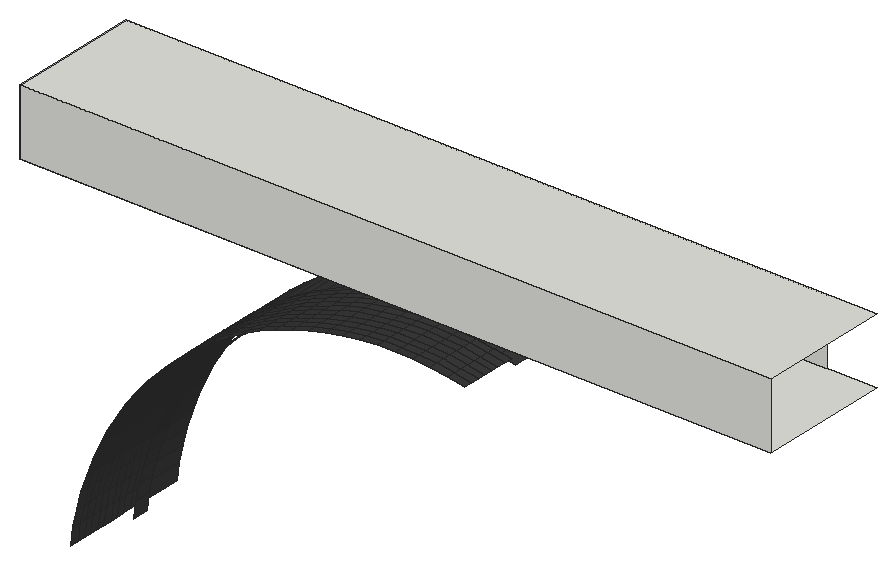
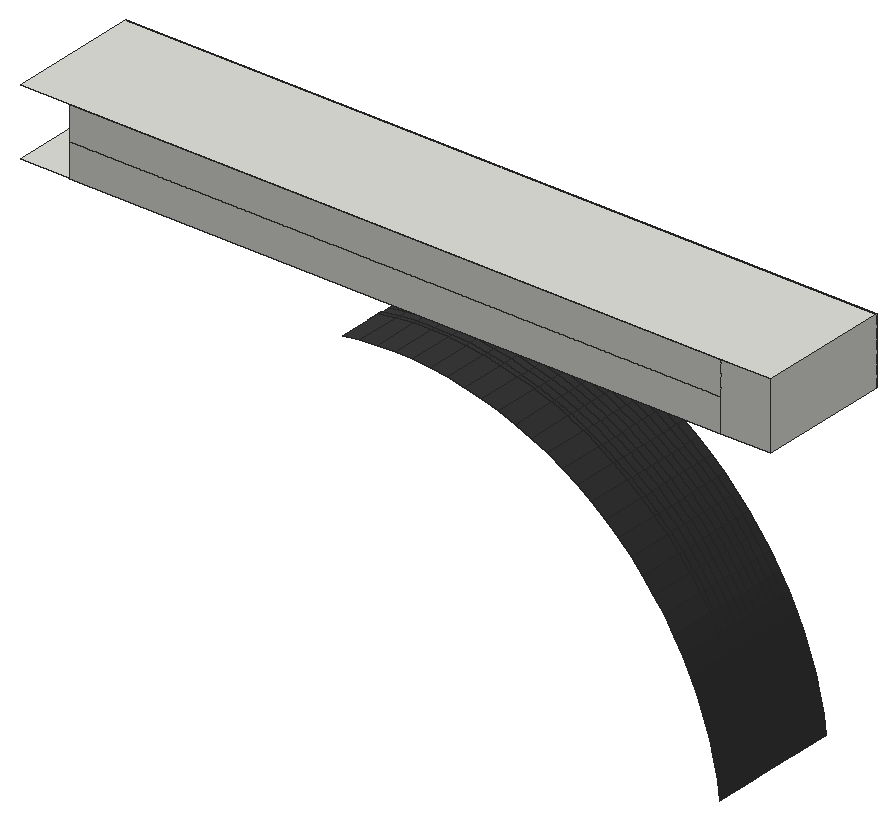
# SketchUp Ruby script. Lengths in inches.
U = 1.inch
M = Sketchup.active_model
def pt(a) = Geom::Point3d.new(a.map { |v| v * U })
def face(e, loops, mat)
  f = e.add_face(loops[0].map { |a| pt(a) })
  loops[1..].each { |l| e.add_face(l.map { |a| pt(a) }).erase! }
  f.material = f.back_material = mat if mat
  f
end
# faces: each face lists its corners as indices into pts; further lists are holes
def faces(e, pts, list, mat = nil) = list.each { |f| face(e, (f[0].is_a?(Array) ? f : [f]).map { |l| l.map { |i| pts[i] } }, mat) }
# xy, xz, yz: faces in a plane at the given z, y or x. An outline is a flat list of corners, or four numbers for a rectangle; further outlines are holes
def ring(l) = l.size == 4 ? [[l[0], l[1]], [l[2], l[1]], [l[2], l[3]], [l[0], l[3]]] : l.each_slice(2).to_a
def flat(e, list, mat, &to3) = list.each { |f| face(e, (f[0].is_a?(Array) ? f : [f]).map { |l| ring(l).map { |u, v| to3.(u, v) } }, mat) }
def xy(e, z, list, mat = nil) = flat(e, list, mat) { |x, y| [x, y, z] }
def xz(e, y, list, mat = nil) = flat(e, list, mat) { |x, z| [x, y, z] }
def yz(e, x, list, mat = nil) = flat(e, list, mat) { |y, z| [x, y, z] }
def lines(e, pts, list) = list.each { |a, b| e.add_line(pt(pts[a]), pt(pts[b])) }
# prism: a flat outline (further loops are holes) pulled along v
def prism(e, loops, v, mat = nil)
  f = face(e, loops, mat); d = Geom::Vector3d.new(v.map { |x| x * U })
  f.pushpull(f.normal.samedirection?(d) ? d.length : -d.length)
end
def box(e, o, s, mat = nil) = prism(e, [[o, [o[0] + s[0], o[1], o[2]], [o[0] + s[0], o[1] + s[1], o[2]], [o[0], o[1] + s[1], o[2]]]], [0, 0, s[2]], mat)
def at(x, y, z, deg = 0) = Geom::Transformation.translation(pt([x, y, z])) * Geom::Transformation.rotation(ORIGIN, Z_AXIS, deg.degrees)
def axes(o, x, y, z) = Geom::Transformation.new([*x, 0, *y, 0, *z, 0, *pt(o).to_a, 1])
def part(name) = M.definitions.add(name)
# library, detail: a bought-in or finely detailed component or shape, given as its bounding box
def library(name, o, s) = part(name).tap { |d| box(d.entities, o, s) }
def detail(e, o, s) = box(e.add_group.entities, o, s)
def put(e, d, t, mat = nil) = e.add_instance(d, t).tap { |i| i.material = mat if mat }
def group(e, t, mat = nil) = e.add_group.tap { |g| g.transformation = t; g.material = mat if mat }.entities
root = M.entities
M.materials.add("[Color M07]").color = [58, 58, 58]
xy(root,373.6875,[[18.46,0,154.46,24]])
xy(root,385.6875,[[18.46,0,154.46,24]])
xz(root,0,[[18.46,373.6875,154.46,385.6875]])
xz(root,24,[[18.46,373.6875,27.46,385.6875],[27.46,373.6875,145.46,379.6875],[27.46,379.6875,145.46,385.6875]])
yz(root,18.46,[[0,373.6875,24,385.6875]])
p = [[29.42,14.875,313.82],[29.87,14.875,316.87],[29.87,12,316.87],[29.42,12,313.82],[27.6,0,314.03],[27.6,1.5,314.03],
  [28.06,1.5,317.1875],[28.06,0,317.1875],[27.6,3,314.03],[28.06,3,317.1875],[27.6,4.5,314.03],[28.06,4.5,317.1875],
  [27.6,6,314.03],[28.06,6,317.1875],[27.6,7.5,314.03],[28.06,7.5,317.1875],[27.6,9,314.03],[28.06,9,317.1875],
  [27.6,10.5,314.03],[28.06,10.5,317.1875],[27.6,12,314.03],[28.06,12,317.1875],[27.6,13.5,314.03],[28.06,13.5,317.1875],
  [27.6,15,314.03],[28.06,15,317.1875],[27.6,15.8125,314.03],[28.06,15.8125,317.1875],[28.06,24,317.1875],[27.6,24,314.03],
  [30.48,14.875,319.9],[30.48,12,319.9],[28.7,1.5,320.31],[28.7,0,320.31],[28.7,3,320.31],[28.7,4.5,320.31],
  [28.7,6,320.31],[28.7,7.5,320.31],[28.7,9,320.31],[28.7,10.5,320.31],[28.7,12,320.31],[28.7,13.5,320.31],
  [28.7,15,320.31],[28.7,15.8125,320.31],[28.7,24,320.31],[31.26,14.875,322.89],[31.26,12,322.89],[29.5,1.5,323.39],
  [29.5,0,323.39],[29.5,3,323.39],[29.5,4.5,323.39],[29.5,6,323.39],[29.5,7.5,323.39],[29.5,9,323.39],
  [29.5,10.5,323.39],[29.5,12,323.39],[29.5,13.5,323.39],[29.5,15,323.39],[29.5,15.8125,323.39],[29.5,24,323.39],
  [32.19,14.875,325.83],[32.19,12,325.83],[30.46,1.5,326.43],[30.46,0,326.43],[30.46,3,326.43],[30.46,4.5,326.43],
  [30.46,6,326.43],[30.46,7.5,326.43],[30.46,9,326.43],[30.46,10.5,326.43],[30.46,12,326.43],[30.46,13.5,326.43],
  [30.46,15,326.43],[30.46,15.8125,326.43],[30.46,24,326.43],[33.28,14.875,328.72],[33.28,12,328.72],[31.59,1.5,329.41],
  [31.59,0,329.41],[31.59,3,329.41],[31.59,4.5,329.41],[31.59,6,329.41],[31.59,7.5,329.41],[31.59,9,329.41],
  [31.59,10.5,329.41],[31.59,12,329.41],[31.59,13.5,329.41],[31.59,15,329.41],[31.59,15.8125,329.41],[31.59,24,329.41],
  [34.53,14.875,331.54],[34.53,12,331.54],[32.875,1.5,332.33],[32.875,0,332.33],[32.875,3,332.33],[32.875,4.5,332.33],
  [32.875,6,332.33],[32.875,7.5,332.33],[32.875,9,332.33],[32.875,10.5,332.33],[32.875,12,332.33],[32.875,13.5,332.33],
  [32.875,15,332.33],[32.875,15.8125,332.33],[32.875,24,332.33],[35.92,14.875,334.3],[35.92,12,334.3],[34.3125,1.5,335.17],
  [34.3125,0,335.17],[34.3125,3,335.17],[34.3125,4.5,335.17],[34.3125,6,335.17],[34.3125,7.5,335.17],[34.3125,9,335.17],
  [34.3125,10.5,335.17],[34.3125,12,335.17],[34.3125,13.5,335.17],[34.3125,15,335.17],[34.3125,15.8125,335.17],[34.3125,24,335.17],
  [37.47,14.875,336.97],[37.47,12,336.97],[35.9,1.5,337.93],[35.9,0,337.93],[35.9,3,337.93],[35.9,4.5,337.93],
  [35.9,6,337.93],[35.9,7.5,337.93],[35.9,9,337.93],[35.9,10.5,337.93],[35.9,12,337.93],[35.9,13.5,337.93],
  [35.9,15,337.93],[35.9,15.8125,337.93],[35.9,24,337.93],[39.15,14.875,339.5625],[39.15,12,339.5625],[37.64,1.5,340.6],
  [37.64,0,340.6],[37.64,3,340.6],[37.64,4.5,340.6],[37.64,6,340.6],[37.64,7.5,340.6],[37.64,9,340.6],
  [37.64,10.5,340.6],[37.64,12,340.6],[37.64,13.5,340.6],[37.64,15,340.6],[37.64,15.8125,340.6],[37.64,24,340.6],
  [40.97,14.875,342.06],[40.97,12,342.06],[39.52,1.5,343.17],[39.52,0,343.17],[39.52,3,343.17],[39.52,4.5,343.17],
  [39.52,6,343.17],[39.52,7.5,343.17],[39.52,9,343.17],[39.52,10.5,343.17],[39.52,12,343.17],[39.52,13.5,343.17],
  [39.52,15,343.17],[39.52,15.8125,343.17],[39.52,24,343.17],[42.92,14.875,344.45],[42.92,12,344.45],[41.53,1.5,345.64],
  [41.53,0,345.64],[41.53,3,345.64],[41.53,4.5,345.64],[41.53,6,345.64],[41.53,7.5,345.64],[41.53,9,345.64],
  [41.53,10.5,345.64],[41.53,12,345.64],[41.53,13.5,345.64],[41.53,15,345.64],[41.53,15.8125,345.64],[41.53,24,345.64],
  [45,14.875,346.74],[45,12,346.74],[43.67,1.5,348],[43.67,0,348],[43.67,3,348],[43.67,4.5,348],
  [43.67,6,348],[43.67,7.5,348],[43.67,9,348],[43.67,10.5,348],[43.67,12,348],[43.67,13.5,348],
  [43.67,15,348],[43.67,15.8125,348],[43.67,24,348],[47.19,14.875,348.91],[47.19,12,348.91],[45.94,1.5,350.24],
  [45.94,0,350.24],[45.94,3,350.24],[45.94,4.5,350.24],[45.94,6,350.24],[45.94,7.5,350.24],[45.94,9,350.24],
  [45.94,10.5,350.24],[45.94,12,350.24],[45.94,13.5,350.24],[45.94,15,350.24],[45.94,15.8125,350.24],[45.94,24,350.24],
  [48.35,14.875,349.93],[49.5,14.875,350.95],[49.5,12,350.95],[48.35,12,349.93],[48.32,1.5,352.36],[48.32,0,352.36],
  [48.32,3,352.36],[48.32,4.5,352.36],[48.32,6,352.36],[48.32,7.5,352.36],[48.32,9,352.36],[48.32,10.5,352.36],
  [48.32,12,352.36],[48.32,13.5,352.36],[48.32,15,352.36],[48.32,15.8125,352.36],[48.32,24,352.36],[51.92,14.875,352.875],
  [51.92,12,352.875],[50.82,1.5,354.34],[50.82,0,354.34],[50.82,3,354.34],[50.82,4.5,354.34],[50.82,6,354.34],
  [50.82,7.5,354.34],[50.82,9,354.34],[50.82,10.5,354.34],[50.82,12,354.34],[50.82,13.5,354.34],[50.82,15,354.34],
  [50.82,15.8125,354.34],[50.82,24,354.34],[54.44,14.875,354.67],[54.44,12,354.67],[53.42,1.5,356.1875],[53.42,0,356.1875],
  [53.42,3,356.1875],[53.42,4.5,356.1875],[53.42,6,356.1875],[53.42,7.5,356.1875],[53.42,9,356.1875],[53.42,10.5,356.1875],
  [53.42,12,356.1875],[53.42,13.5,356.1875],[53.42,15,356.1875],[53.42,15.8125,356.1875],[53.42,24,356.1875],[57.04,14.875,356.32],
  [57.04,12,356.32],[56.11,1.5,357.89],[56.11,0,357.89],[56.11,3,357.89],[56.11,4.5,357.89],[56.11,6,357.89],
  [56.11,7.5,357.89],[56.11,9,357.89],[56.11,10.5,357.89],[56.11,12,357.89],[56.11,13.5,357.89],[56.11,15,357.89],
  [56.11,15.8125,357.89],[56.11,24,357.89],[59.74,14.875,357.83],[59.74,12,357.83],[62.51,14.875,359.19],[62.51,12,359.19],
  [58.89,1.5,359.45],[58.89,0,359.45],[58.89,3,359.45],[58.89,4.5,359.45],[58.89,6,359.45],[58.89,7.5,359.45],
  [58.89,9,359.45],[58.89,10.5,359.45],[58.89,12,359.45],[58.89,13.5,359.45],[58.89,15,359.45],[58.89,15.8125,359.45],
  [58.89,24,359.45],[65.35,14.875,360.4],[65.35,12,360.4],[61.75,1.5,360.85],[61.75,0,360.85],[61.75,3,360.85],
  [61.75,4.5,360.85],[61.75,6,360.85],[61.75,7.5,360.85],[61.75,9,360.85],[61.75,10.5,360.85],[61.75,12,360.85],
  [61.75,13.5,360.85],[61.75,15,360.85],[61.75,15.8125,360.85],[61.75,24,360.85],[68.25,14.875,361.46],[68.25,12,361.46],
  [64.68,1.5,362.1],[64.68,0,362.1],[64.68,3,362.1],[64.68,4.5,362.1],[64.68,6,362.1],[64.68,7.5,362.1],
  [64.68,9,362.1],[64.68,10.5,362.1],[64.68,12,362.1],[64.68,13.5,362.1],[64.68,15,362.1],[64.68,15.8125,362.1],
  [64.68,24,362.1],[71.21,14.875,362.36],[71.21,12,362.36],[67.67,1.5,363.19],[67.67,0,363.19],[67.67,3,363.19],
  [67.67,4.5,363.19],[67.67,6,363.19],[67.67,7.5,363.19],[67.67,9,363.19],[67.67,10.5,363.19],[67.67,12,363.19],
  [67.67,13.5,363.19],[67.67,15,363.19],[67.67,15.8125,363.19],[67.67,24,363.19],[74.2,14.875,363.1],[74.2,12,363.1],
  [75.72,14.875,363.39],[75.72,12,363.39],[95.6875,14.875,363.67],[98.72,14.875,363.1],[98.72,12,363.1],[95.6875,12,363.67],
  [70.72,1.5,364.12],[70.72,0,364.12],[70.72,3,364.12],[70.72,4.5,364.12],[70.72,6,364.12],[70.72,7.5,364.12],
  [70.72,9,364.12],[70.72,10.5,364.12],[70.72,12,364.12],[70.72,13.5,364.12],[70.72,15,364.12],[70.72,15.8125,364.12],
  [70.72,24,364.12],[77.24,14.875,363.67],[80.3,14.875,364.09],[80.3,12,364.09],[77.24,12,363.67],[92.625,14.875,364.09],
  [92.625,12,364.09],[73.8125,1.5,364.88],[73.8125,0,364.88],[73.8125,3,364.88],[73.8125,4.5,364.88],[73.8125,6,364.88],
  [73.8125,7.5,364.88],[73.8125,9,364.88],[73.8125,10.5,364.88],[73.8125,12,364.88],[73.8125,13.5,364.88],[83.375,14.875,364.34],
  [83.375,12,364.34],[89.55,14.875,364.34],[89.55,12,364.34],[73.8125,15,364.88],[73.8125,15.8125,364.88],[73.8125,24,364.88],
  [86.46,14.875,364.42],[86.46,12,364.42],[76.94,1.5,365.48],[76.94,0,365.48],[95.98,0,365.48],[95.98,1.5,365.48],
  [99.11,1.5,364.88],[99.11,0,364.88],[76.94,3,365.48],[95.98,3,365.48],[99.11,3,364.88],[76.94,4.5,365.48],
  [95.98,4.5,365.48],[99.11,4.5,364.88],[76.94,6,365.48],[95.98,6,365.48],[99.11,6,364.88],[76.94,7.5,365.48],
  [95.98,7.5,365.48],[99.11,7.5,364.88],[76.94,9,365.48],[95.98,9,365.48],[99.11,9,364.88],[76.94,10.5,365.48],
  [95.98,10.5,365.48],[99.11,10.5,364.88],[76.94,12,365.48],[76.94,13.5,365.48],[76.94,15,365.48],[76.94,15.8125,365.48],
  [76.94,24,365.48],[80.1,1.5,365.91],[80.1,0,365.91],[92.82,0,365.91],[92.82,1.5,365.91],[80.1,3,365.91],
  [92.82,3,365.91],[80.1,4.5,365.91],[92.82,4.5,365.91],[80.1,6,365.91],[92.82,6,365.91],[80.1,7.5,365.91],
  [92.82,7.5,365.91],[80.1,9,365.91],[92.82,9,365.91],[80.1,10.5,365.91],[92.82,10.5,365.91],[80.1,12,365.91],
  [92.82,12,365.91],[95.98,12,365.48],[80.1,13.5,365.91],[92.82,13.5,365.91],[95.98,13.5,365.48],[80.1,15,365.91],
  [92.82,15,365.91],[95.98,15,365.48],[80.1,15.8125,365.91],[92.82,15.8125,365.91],[95.98,15.8125,365.48],[80.1,24,365.91],
  [95.98,24,365.48],[92.82,24,365.91],[83.28,1.5,366.16],[83.28,0,366.16],[89.65,0,366.16],[89.65,1.5,366.16],
  [83.28,3,366.16],[89.65,3,366.16],[83.28,4.5,366.16],[89.65,4.5,366.16],[83.28,6,366.16],[89.65,6,366.16],
  [83.28,7.5,366.16],[89.65,7.5,366.16],[83.28,9,366.16],[89.65,9,366.16],[83.28,10.5,366.16],[89.65,10.5,366.16],
  [83.28,12,366.16],[89.65,12,366.16],[83.28,13.5,366.16],[89.65,13.5,366.16],[83.28,15,366.16],[89.65,15,366.16],
  [83.28,15.8125,366.16],[89.65,15.8125,366.16],[83.28,24,366.16],[89.65,24,366.16],[86.46,1.5,366.25],[86.46,0,366.25],
  [86.46,3,366.25],[86.46,4.5,366.25],[86.46,6,366.25],[86.46,7.5,366.25],[86.46,9,366.25],[86.46,10.5,366.25],
  [86.46,12,366.25],[86.46,13.5,366.25],[86.46,15,366.25],[86.46,15.8125,366.25],[86.46,24,366.25]]
faces(root,p,[[0,1,2,3],[4,5,6,7],[5,8,9,6],[8,10,11,9],[10,12,13,11],[12,14,15,13],[14,16,17,15],[16,18,19,17],
  [18,20,21,19],[22,20,21,23],[24,22,23,25],[26,27,25,24],[28,27,26,29],[1,30,31,2],[7,6,32,33],[6,9,34,32],
  [9,11,35,34],[11,13,36,35],[13,15,37,36],[15,17,38,37],[17,19,39,38],[19,21,40,39],[23,21,40,41],[25,23,41,42],
  [27,43,42,25],[44,43,27,28],[30,45,46,31],[33,32,47,48],[32,34,49,47],[34,35,50,49],[35,36,51,50],[36,37,52,51],
  [37,38,53,52],[38,39,54,53],[39,40,55,54],[41,40,55,56],[42,41,56,57],[43,58,57,42],[59,58,43,44],[45,60,61,46],
  [48,47,62,63],[47,49,64,62],[49,50,65,64],[50,51,66,65],[51,52,67,66],[52,53,68,67],[53,54,69,68],[54,55,70,69],
  [56,55,70,71],[57,56,71,72],[58,73,72,57],[74,73,58,59],[60,75,76,61],[63,62,77,78],[62,64,79,77],[64,65,80,79],
  [65,66,81,80],[66,67,82,81],[67,68,83,82],[68,69,84,83],[69,70,85,84],[71,70,85,86],[72,71,86,87],[73,88,87,72],
  [89,88,73,74],[75,90,91,76],[78,77,92,93],[77,79,94,92],[79,80,95,94],[80,81,96,95],[81,82,97,96],[82,83,98,97],
  [83,84,99,98],[84,85,100,99],[86,85,100,101],[87,86,101,102],[88,103,102,87],[104,103,88,89],[90,105,106,91],[93,92,107,108],
  [92,94,109,107],[94,95,110,109],[95,96,111,110],[96,97,112,111],[97,98,113,112],[98,99,114,113],[99,100,115,114],[101,100,115,116],
  [102,101,116,117],[103,118,117,102],[119,118,103,104],[105,120,121,106],[108,107,122,123],[107,109,124,122],[109,110,125,124],[110,111,126,125],
  [111,112,127,126],[112,113,128,127],[113,114,129,128],[114,115,130,129],[116,115,130,131],[117,116,131,132],[118,133,132,117],[134,133,118,119],
  [120,135,136,121],[123,122,137,138],[122,124,139,137],[124,125,140,139],[125,126,141,140],[126,127,142,141],[127,128,143,142],[128,129,144,143],
  [129,130,145,144],[131,130,145,146],[132,131,146,147],[133,148,147,132],[149,148,133,134],[135,150,151,136],[138,137,152,153],[137,139,154,152],
  [139,140,155,154],[140,141,156,155],[141,142,157,156],[142,143,158,157],[143,144,159,158],[144,145,160,159],[146,145,160,161],[147,146,161,162],
  [148,163,162,147],[164,163,148,149],[150,165,166,151],[153,152,167,168],[152,154,169,167],[154,155,170,169],[155,156,171,170],[156,157,172,171],
  [157,158,173,172],[158,159,174,173],[159,160,175,174],[161,160,175,176],[162,161,176,177],[163,178,177,162],[179,178,163,164],[165,180,181,166],
  [168,167,182,183],[167,169,184,182],[169,170,185,184],[170,171,186,185],[171,172,187,186],[172,173,188,187],[173,174,189,188],[174,175,190,189],
  [176,175,190,191],[177,176,191,192],[178,193,192,177],[194,193,178,179],[180,195,196,181],[183,182,197,198],[182,184,199,197],[184,185,200,199],
  [185,186,201,200],[186,187,202,201],[187,188,203,202],[188,189,204,203],[189,190,205,204],[191,190,205,206],[192,191,206,207],[193,208,207,192],
  [209,208,193,194],[210,211,212,213],[198,197,214,215],[197,199,216,214],[199,200,217,216],[200,201,218,217],[201,202,219,218],[202,203,220,219],
  [203,204,221,220],[204,205,222,221],[206,205,222,223],[207,206,223,224],[208,225,224,207],[226,225,208,209],[211,227,228,212],[215,214,229,230],
  [214,216,231,229],[216,217,232,231],[217,218,233,232],[218,219,234,233],[219,220,235,234],[220,221,236,235],[221,222,237,236],[223,222,237,238],
  [224,223,238,239],[225,240,239,224],[241,240,225,226],[227,242,243,228],[230,229,244,245],[229,231,246,244],[231,232,247,246],[232,233,248,247],
  [233,234,249,248],[234,235,250,249],[235,236,251,250],[236,237,252,251],[238,237,252,253],[239,238,253,254],[240,255,254,239],[256,255,240,241],
  [242,257,258,243],[245,244,259,260],[244,246,261,259],[246,247,262,261],[247,248,263,262],[248,249,264,263],[249,250,265,264],[250,251,266,265],
  [251,252,267,266],[253,252,267,268],[254,253,268,269],[255,270,269,254],[271,270,255,256],[257,272,273,258],[272,274,275,273],[260,259,276,277],
  [259,261,278,276],[261,262,279,278],[262,263,280,279],[263,264,281,280],[264,265,282,281],[265,266,283,282],[266,267,284,283],[268,267,284,285],
  [269,268,285,286],[270,287,286,269],[288,287,270,271],[274,289,290,275],[277,276,291,292],[276,278,293,291],[278,279,294,293],[279,280,295,294],
  [280,281,296,295],[281,282,297,296],[282,283,298,297],[283,284,299,298],[285,284,299,300],[286,285,300,301],[287,302,301,286],[303,302,287,288],
  [289,304,305,290],[292,291,306,307],[291,293,308,306],[293,294,309,308],[294,295,310,309],[295,296,311,310],[296,297,312,311],[297,298,313,312],
  [298,299,314,313],[300,299,314,315],[301,300,315,316],[302,317,316,301],[318,317,302,303],[304,319,320,305],[307,306,321,322],[306,308,323,321],
  [308,309,324,323],[309,310,325,324],[310,311,326,325],[311,312,327,326],[312,313,328,327],[313,314,329,328],[315,314,329,330],[316,315,330,331],
  [317,332,331,316],[333,332,317,318],[319,334,335,320],[334,336,337,335],[338,339,340,341],[322,321,342,343],[321,323,344,342],[323,324,345,344],
  [324,325,346,345],[325,326,347,346],[326,327,348,347],[327,328,349,348],[328,329,350,349],[330,329,350,351],[331,330,351,352],[332,353,352,331],
  [354,353,332,333],[355,356,357,358],[359,338,341,360],[343,342,361,362],[342,344,363,361],[344,345,364,363],[345,346,365,364],[346,347,366,365],
  [347,348,367,366],[348,349,368,367],[349,350,369,368],[351,350,369,370],[356,371,372,357],[373,359,360,374],[352,351,370,375],[353,376,375,352],
  [377,376,353,354],[371,378,379,372],[378,373,374,379],[362,361,380,381],[382,383,384,385],[361,363,386,380],[383,387,388,384],[363,364,389,386],
  [387,390,391,388],[364,365,392,389],[390,393,394,391],[365,366,395,392],[393,396,397,394],[366,367,398,395],[396,399,400,397],[367,368,401,398],
  [399,402,403,400],[368,369,404,401],[370,369,404,405],[375,370,405,406],[376,407,406,375],[408,407,376,377],[381,380,409,410],[411,412,383,382],
  [380,386,413,409],[412,414,387,383],[386,389,415,413],[414,416,390,387],[389,392,417,415],[416,418,393,390],[392,395,419,417],[418,420,396,393],
  [395,398,421,419],[420,422,399,396],[398,401,423,421],[422,424,402,399],[401,404,425,423],[424,426,427,402],[405,404,425,428],[429,426,427,430],
  [406,405,428,431],[432,429,430,433],[407,434,431,406],[435,436,433,432],[437,434,407,408],[438,436,435,439],[410,409,440,441],[442,443,412,411],
  [409,413,444,440],[443,445,414,412],[413,415,446,444],[445,447,416,414],[415,417,448,446],[447,449,418,416],[417,419,450,448],[449,451,420,418],
  [419,421,452,450],[451,453,422,420],[421,423,454,452],[453,455,424,422],[423,425,456,454],[455,457,426,424],[428,425,456,458],[459,457,426,429],
  [431,428,458,460],[461,459,429,432],[434,462,460,431],[463,435,432,461],[464,462,434,437],[439,435,463,465],[441,440,466,467],[467,466,443,442],
  [440,444,468,466],[466,468,445,443],[444,446,469,468],[468,469,447,445],[446,448,470,469],[469,470,449,447],[448,450,471,470],[470,471,451,449],
  [450,452,472,471],[471,472,453,451],[452,454,473,472],[472,473,455,453],[454,456,474,473],[473,474,457,455],[458,456,474,475],[475,474,457,459],
  [460,458,475,476],[476,475,459,461],[462,477,476,460],[477,463,461,476],[478,477,462,464],[465,463,477,478]],"[Color M07]")
